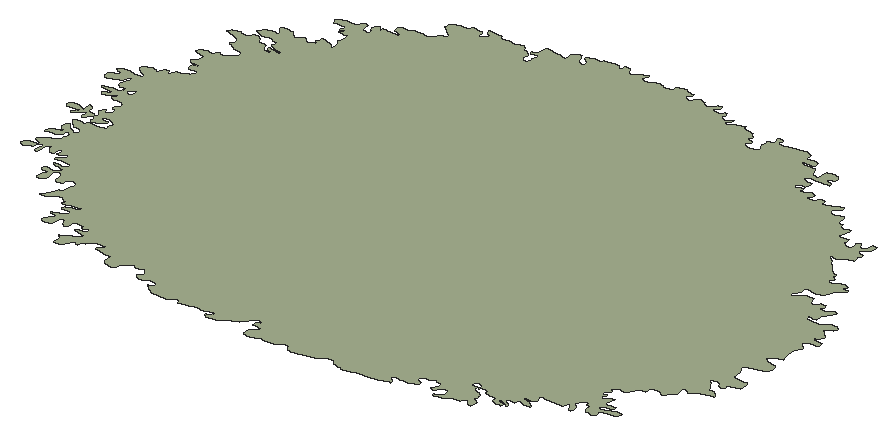
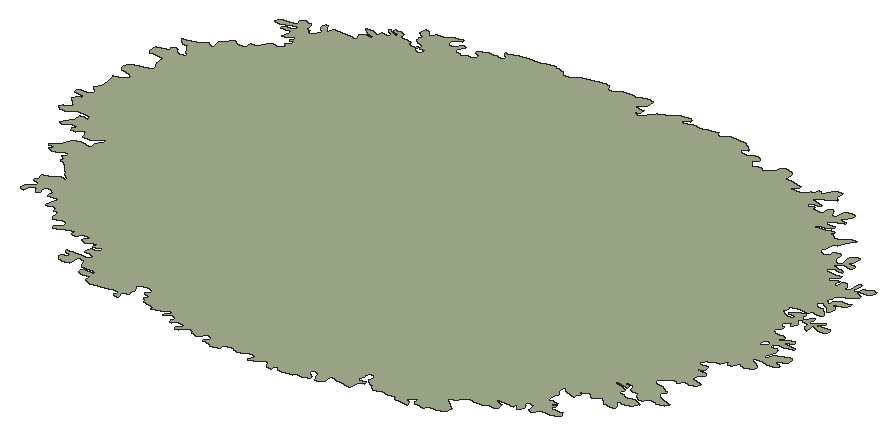
# SketchUp Ruby script. Lengths in inches.
U = 1.inch
M = Sketchup.active_model
def pt(a) = Geom::Point3d.new(a.map { |v| v * U })
def face(e, loops, mat)
  f = e.add_face(loops[0].map { |a| pt(a) })
  loops[1..].each { |l| e.add_face(l.map { |a| pt(a) }).erase! }
  f.material = f.back_material = mat if mat
  f
end
# faces: each face lists its corners as indices into pts; further lists are holes
def faces(e, pts, list, mat = nil) = list.each { |f| face(e, (f[0].is_a?(Array) ? f : [f]).map { |l| l.map { |i| pts[i] } }, mat) }
# xy, xz, yz: faces in a plane at the given z, y or x. An outline is a flat list of corners, or four numbers for a rectangle; further outlines are holes
def ring(l) = l.size == 4 ? [[l[0], l[1]], [l[2], l[1]], [l[2], l[3]], [l[0], l[3]]] : l.each_slice(2).to_a
def flat(e, list, mat, &to3) = list.each { |f| face(e, (f[0].is_a?(Array) ? f : [f]).map { |l| ring(l).map { |u, v| to3.(u, v) } }, mat) }
def xy(e, z, list, mat = nil) = flat(e, list, mat) { |x, y| [x, y, z] }
def xz(e, y, list, mat = nil) = flat(e, list, mat) { |x, z| [x, y, z] }
def yz(e, x, list, mat = nil) = flat(e, list, mat) { |y, z| [x, y, z] }
def lines(e, pts, list) = list.each { |a, b| e.add_line(pt(pts[a]), pt(pts[b])) }
# prism: a flat outline (further loops are holes) pulled along v
def prism(e, loops, v, mat = nil)
  f = face(e, loops, mat); d = Geom::Vector3d.new(v.map { |x| x * U })
  f.pushpull(f.normal.samedirection?(d) ? d.length : -d.length)
end
def box(e, o, s, mat = nil) = prism(e, [[o, [o[0] + s[0], o[1], o[2]], [o[0] + s[0], o[1] + s[1], o[2]], [o[0], o[1] + s[1], o[2]]]], [0, 0, s[2]], mat)
def at(x, y, z, deg = 0) = Geom::Transformation.translation(pt([x, y, z])) * Geom::Transformation.rotation(ORIGIN, Z_AXIS, deg.degrees)
def axes(o, x, y, z) = Geom::Transformation.new([*x, 0, *y, 0, *z, 0, *pt(o).to_a, 1])
def part(name) = M.definitions.add(name)
# library, detail: a bought-in or finely detailed component or shape, given as its bounding box
def library(name, o, s) = part(name).tap { |d| box(d.entities, o, s) }
def detail(e, o, s) = box(e.add_group.entities, o, s)
def put(e, d, t, mat = nil) = e.add_instance(d, t).tap { |i| i.material = mat if mat }
def group(e, t, mat = nil) = e.add_group.tap { |g| g.transformation = t; g.material = mat if mat }.entities
root = M.entities
M.materials.add("Boxwoodplan").color = [166, 177, 144]
xy(root,9.058,[[[52.292,67.129,52.181,67.133,52.086,67.159,52.03,67.215,52.028,67.317,52.054,67.382,52.118,67.445,52.167,67.509,52.225,67.606,52.039,67.635,51.949,67.644,51.969,67.732,52.055,67.79,52.086,67.8,52.081,67.846,51.992,67.877,51.876,67.837,51.779,67.706,51.636,67.551,51.475,67.464,51.37,67.441,51.309,67.416,51.293,67.373,51.149,67.281,50.955,67.251,50.866,67.26,50.786,67.306,50.786,67.328,50.831,67.359,50.922,67.437,50.99,67.483,50.901,67.498,50.788,67.48,50.668,67.436,50.572,67.445,50.475,67.454,50.378,67.447,50.251,67.403,50.051,67.356,49.962,67.349,49.924,67.443,49.916,67.465,49.849,67.473,49.76,67.454,49.591,67.336,49.391,67.328,49.161,67.353,48.994,67.446,48.853,67.61,49.036,67.702,48.936,67.756,48.8,67.772,48.674,67.749,48.602,67.697,48.521,67.672,48.405,67.738,48.363,67.806,48.451,67.847,48.477,67.907,48.482,67.957,48.441,68.009,48.369,68.085,48.283,68.117,48.196,68.064,48.13,68.038,48.074,68.08,48.057,68.103,48.033,68.121,48.004,68.111,47.924,68.058,47.853,68.01,47.777,67.923,47.765,67.79,47.694,67.749,47.644,67.723,47.584,67.725,47.485,67.746,47.398,67.793,47.354,67.861,47.346,67.951,47.355,68.018,47.368,68.04,47.349,68.08,47.135,68.1,47.203,68.135,47.177,68.136,47.084,68.13,46.914,68.146,46.837,68.173,46.82,68.206,46.835,68.224,46.96,68.314,46.958,68.371,46.873,68.393,46.714,68.39,46.583,68.319,46.486,68.233,46.411,68.199,46.364,68.172,46.363,68.154,46.399,68.101,46.383,68.046,46.313,68.081,46.249,68.121,46.188,68.072,46.166,68.017,46.134,67.904,46.087,67.855,46.014,67.822,45.923,67.816,45.853,67.841,45.834,67.874,45.841,67.892,45.862,67.932,45.884,67.991,45.853,68.048,45.752,68.149,45.866,68.229,45.927,68.269,46.007,68.285,46.074,68.315,46.129,68.37,46.214,68.476,46.142,68.503,46.0625,68.511,45.93,68.53,45.892,68.565,45.899,68.584,45.974,68.62,46.136,68.657,46.178,68.709,46.173,68.748,46.147,68.764,45.997,68.711,45.951,68.732,45.952,68.752,45.975,68.814,45.814,68.825,45.733,68.833,45.679,68.826,45.672,68.806,45.656,68.71,45.641,68.642,45.599,68.591,45.552,68.578,45.533,68.594,45.474,68.639,45.429,68.757,45.39,68.783,45.363,68.784,45.309,68.777,45.302,68.757,45.3,68.641,45.246,68.523,45.185,68.449,45.105,68.419,45.026,68.422,44.98,68.448,44.947,68.506,44.947,68.564,45.001,68.677,45.115,68.784,45.135,68.803,45.122,68.823,45.095,68.829,45.015,68.847,44.934,68.86,44.907,68.875,44.914,68.895,44.934,68.914,45.083,68.982,45.245,69.005,45.287,69.108,45.26,69.169,45.213,69.191,45.186,69.187,45.023,69.168,44.982,69.2,44.989,69.22,45.016,69.279,45.174,69.334,45.346,69.403,45.394,69.442,45.381,69.463,45.284,69.436,45.113,69.417,44.969,69.372,44.88,69.386,44.853,69.392,44.859,69.412,44.88,69.426,44.935,69.47,44.907,69.507,44.88,69.503,44.797,69.511,44.742,69.56,44.728,69.601,44.701,69.597,44.618,69.575,44.461,69.489,44.312,69.413,44.238,69.38,44.183,69.392,44.196,69.412,44.215,69.452,44.242,69.469,44.266,69.55,44.316,69.65,44.348,69.759,44.399,69.812,44.472,69.852,44.516,69.972,44.538,70.112,44.558,70.227,44.554,70.285,44.509,70.321,44.428,70.335,44.342,70.335,44.268,70.31,44.258,70.245,44.259,70.184,44.226,70.124,44.138,70.087,44.081,70.096,44.043,70.155,44.032,70.216,44.006,70.337,44.001,70.4,43.96,70.453,43.933,70.475,43.895,70.491,43.836,70.479,43.802,70.46,43.8,70.428,43.792,70.366,43.795,70.229,43.82,70.167,43.812,70.103,43.761,70.038,43.713,70.01,43.675,69.998,43.637,70.003,43.595,70.011,43.577,70.039,43.573,70.166,43.594,70.223,43.639,70.276,43.655,70.306,43.647,70.334,43.59,70.34,43.508,70.346,43.471,70.362,43.448,70.39,43.445,70.453,43.46,70.483,43.495,70.499,43.667,70.472,43.746,70.497,43.795,70.526,43.856,70.573,43.869,70.636,43.846,70.662,43.802,70.664,43.725,70.67,43.633,70.681,43.532,70.717,43.513,70.746,43.519,70.76,43.538,70.763,43.598,70.775,43.773,70.761,43.863,70.787,43.875,70.844,43.849,70.907,43.777,70.946,43.698,70.953,43.585,70.946,43.485,70.921,43.402,70.939,43.398,70.968,43.418,70.997,43.465,71.054,43.531,71.11,43.584,71.19,43.576,71.224,43.531,71.241,43.466,71.24,43.348,71.14,43.308,71.141,43.274,71.161,43.296,71.22,43.312,71.287,43.269,71.35,43.229,71.366,43.209,71.367,43.203,71.352,43.207,71.306,43.204,71.164,43.163,71.102,43.124,71.108,43.089,71.131,42.991,71.262,42.967,71.327,42.942,71.355,42.927,71.344,42.871,71.293,42.836,71.234,42.856,71.103,42.861,71.037,42.841,70.971,42.791,70.962,42.757,70.978,42.747,71.023,42.767,71.155,42.776,71.233,42.776,71.27,42.761,71.282,42.746,71.272,42.667,71.237,42.627,71.183,42.618,71.12,42.579,71.077,42.442,70.987,42.402,70.977,42.358,70.986,42.278,71.026,42.258,71.056,42.262,71.089,42.295,71.151,42.392,71.237,42.482,71.263,42.572,71.263,42.667,71.267,42.606,71.318,42.455,71.404,42.438,71.466,42.491,71.503,42.583,71.573,42.702,71.635,42.82,71.709,42.856,71.723,42.882,71.746,42.908,71.789,42.911,71.882,42.944,72.003,42.945,72.065,42.924,72.086,42.902,72.095,42.839,72.109,42.806,72.104,42.802,72.088,42.814,71.996,42.772,71.934,42.724,71.899,42.647,71.871,42.576,71.858,42.415,71.833,42.38,71.839,42.367,71.853,42.367,71.86,42.376,71.901,42.393,71.947,42.435,71.995,42.504,72.042,42.563,72.063,42.621,72.065,42.66,72.068,42.68,72.075,42.703,72.096,42.698,72.121,42.644,72.151,42.576,72.207,42.544,72.264,42.54,72.331,42.553,72.382,42.605,72.426,42.631,72.432,42.642,72.425,42.662,72.411,42.705,72.35,42.754,72.304,42.882,72.226,42.956,72.192,42.991,72.177,43.011,72.184,43.035,72.206,43.042,72.222,43.053,72.263,43.038,72.32,42.995,72.366,42.963,72.389,42.929,72.401,42.869,72.401,42.795,72.404,42.752,72.446,42.666,72.519,42.607,72.569,42.568,72.617,42.569,72.646,42.593,72.671,42.649,72.698,42.684,72.703,42.725,72.7,42.785,72.679,42.847,72.677,42.883,72.684,42.917,72.726,42.966,72.757,43.025,72.764,43.096,72.764,43.25,72.771,43.39,72.792,43.423,72.808,43.424,72.826,43.418,72.868,43.406,72.913,43.417,72.957,43.447,73.06,43.434,73.083,43.411,73.097,43.354,73.126,43.301,73.164,43.228,73.192,43.155,73.195,43.105,73.184,43.084,73.17,43.059,73.119,43.064,73.098,43.075,73.093,43.099,73.088,43.25,73.076,43.276,73.071,43.281,73.0625,43.272,73.046,43.232,73.007,43.187,72.964,43.122,72.928,43.06,72.884,42.988,72.849,42.951,72.852,42.931,72.863,42.906,72.9,42.899,72.995,42.882,73.02,42.9,73.034,42.906,73.077,42.9,73.088,42.889,73.088,42.874,73.087,42.848,73.083,42.816,73.076,42.798,73.065,42.717,72.97,42.685,72.915,42.654,72.892,42.631,72.895,42.605,72.916,42.596,72.932,42.59,72.973,42.619,73.057,42.624,73.102,42.615,73.13,42.595,73.137,42.557,73.128,42.537,73.114,42.491,73.064,42.369,72.957,42.333,72.932,42.307,72.927,42.27,72.935,42.258,72.951,42.349,73.057,42.412,73.102,42.426,73.129,42.425,73.145,42.416,73.152,42.405,73.148,42.39,73.143,42.359,73.131,42.275,73.108,42.108,73.089,42.035,73.096,41.987,73.121,41.965,73.149,41.964,73.165,41.981,73.217,42.029,73.264,42.089,73.281,42.16,73.284,42.234,73.266,42.362,73.223,42.448,73.197,42.459,73.201,42.459,73.22,42.45,73.239,42.425,73.287,42.424,73.342,42.431,73.407,42.443,73.437,42.46,73.45,42.509,73.413,42.548,73.363,42.575,73.317,42.585,73.255,42.597,73.204,42.612,73.176,42.635,73.175,42.77,73.157,42.843,73.144,42.878,73.14,42.896,73.154,42.911,73.202,42.856,73.244,42.797,73.309,42.78,73.335,42.78,73.352,42.814,73.46,42.844,73.483,42.871,73.489,42.886,73.477,42.895,73.459,42.924,73.414,42.935,73.39,42.947,73.391,42.968,73.404,43.048,73.482,43.065,73.528,43.066,73.579,43.052,73.611,43.031,73.623,42.968,73.646,42.928,73.666,42.92,73.687,42.936,73.736,42.992,73.773,43.026,73.795,43.039,73.816,43.047,73.869,43.045,73.916,42.95,73.992,42.806,74.014,42.744,74.031,42.709,74.013,42.681,74.014,42.612,74.031,42.593,74.058,42.602,74.082,42.728,74.185,42.722,74.217,42.7,74.233,42.655,74.225,42.626,74.216,42.5,74.154,42.46,74.107,42.411,74.063,42.342,74.049,42.314,74.05,42.267,74.102,42.295,74.126,42.3125,74.165,42.344,74.188,42.438,74.22,42.483,74.25,42.472,74.281,42.459,74.283,42.449,74.276,42.423,74.27,42.384,74.273,42.249,74.284,42.102,74.3125,42.078,74.327,42.084,74.347,42.109,74.375,42.322,74.435,42.385,74.434,42.446,74.419,42.506,74.391,42.533,74.393,42.539,74.403,42.588,74.48,42.612,74.495,42.618,74.515,42.618,74.583,42.607,74.593,42.594,74.591,42.536,74.591,42.479,74.585,42.432,74.568,42.408,74.576,42.387,74.596,42.362,74.63,42.342,74.718,42.353,74.806,42.383,74.848,42.389,74.88,42.402,74.923,42.439,74.944,42.435,74.99,42.413,75.026,42.324,75.003,42.306,74.969,42.307,74.95,42.31,74.886,42.23,74.839,42.089,74.745,41.933,74.7,41.849,74.725,41.807,74.778,41.798,74.904,41.926,74.99,42.009,75.003,42.052,75.027,42.076,75.061,42.075,75.081,41.989,75.112,41.916,75.138,41.854,75.194,41.889,75.249,41.965,75.278,42.061,75.312,42.126,75.311,42.305,75.267,42.397,75.246,42.482,75.25,42.533,75.269,42.539,75.289,42.523,75.355,42.462,75.407,42.417,75.415,42.305,75.485,42.258,75.527,42.244,75.564,42.237,75.617,42.237,75.644,42.25,75.659,42.292,75.695,42.343,75.709,42.457,75.741,42.488,75.751,42.528,75.75,42.578,75.746,42.591,75.733,42.606,75.703,42.62,75.689,42.63,75.689,42.658,75.692,42.674,75.704,42.695,75.754,42.723,75.787,42.739,75.81,42.742,75.835,42.758,75.86,42.778,75.872,42.826,75.884,42.865,75.877,42.886,75.833,42.89,75.781,42.907,75.755,42.928,75.754,42.97,75.796,42.995,75.838,43.009,75.942,43.025,75.968,43.057,75.975,43.089,75.974,43.108,75.963,43.129,75.94,43.161,75.94,43.214,75.961,43.258,76.007,43.272,76.032,43.261,76.046,43.321,76.043,43.35,76.046,43.366,76.066,43.371,76.114,43.405,76.155,43.439,76.2,43.385,76.243,43.318,76.272,43.281,76.271,43.248,76.261,43.206,76.249,43.164,76.255,43.142,76.271,43.121,76.295,43.098,76.397,43.111,76.423,43.116,76.439,43.126,76.443,43.231,76.463,43.277,76.472,43.295,76.483,43.285,76.486,43.199,76.514,43.133,76.526,43.105,76.519,43.07,76.52,43.034,76.52,42.998,76.532,42.96,76.582,42.942,76.611,42.942,76.642,42.957,76.663,42.986,76.678,43.017,76.697,43.025,76.725,43.055,76.782,43.082,76.836,43.088,76.89,43.081,76.917,43.041,76.928,42.963,76.954,42.79,77.001,42.754,77.018,42.737,77.042,42.773,77.097,42.817,77.131,42.863,77.159,42.918,77.178,42.97,77.1875,43.023,77.184,43.078,77.16,43.133,77.162,43.16,77.167,43.173,77.187,43.19,77.228,43.227,77.264,43.248,77.282,43.274,77.284,43.343,77.267,43.405,77.256,43.431,77.253,43.455,77.268,43.542,77.336,43.629,77.401,43.683,77.498,43.679,77.542,43.638,77.579,43.521,77.617,43.395,77.647,43.309,77.719,43.251,77.755,43.182,77.776,43.155,77.788,43.141,77.808,43.163,77.855,43.211,77.896,43.209,77.981,43.159,78.06,43.029,78.116,42.741,78.212,42.72,78.246,42.792,78.31,42.913,78.362,43.018,78.367,43.075,78.353,43.119,78.327,43.168,78.317,43.221,78.326,43.282,78.337,43.311,78.368,43.326,78.448,43.343,78.483,43.397,78.482,43.454,78.471,43.502,78.451,43.569,78.392,43.593,78.358,43.607,78.318,43.608,78.249,43.614,78.245,43.623,78.249,43.65,78.262,43.701,78.268,43.79,78.271,43.87,78.235,43.904,78.17,43.929,78.092,43.999,78.047,44.039,78.035,44.057,78.034,44.084,78.043,44.179,78.05,44.196,78.055,44.176,78.071,44.113,78.095,44.061,78.099,44.023,78.118,44.004,78.152,44.001,78.164,44.004,78.184,44.019,78.191,44.054,78.192,44.096,78.185,44.202,78.156,44.317,78.152,44.369,78.159,44.387,78.162,44.413,78.173,44.369,78.203,44.328,78.213,44.242,78.228,44.184,78.242,44.143,78.244,44.121,78.248,44.096,78.263,44.044,78.289,43.997,78.315,43.975,78.348,43.985,78.404,44.014,78.442,44.055,78.471,44.015,78.502,43.96,78.517,43.917,78.52,43.862,78.528,43.831,78.555,43.813,78.591,43.799,78.6,43.77,78.599,43.654,78.571,43.602,78.557,43.553,78.559,43.505,78.562,43.456,78.578,43.408,78.595,43.368,78.602,43.282,78.65,43.307,78.662,43.309,78.669,43.32,78.709,43.336,78.745,43.362,78.782,43.393,78.814,43.437,78.839,43.49,78.862,43.535,78.873,43.641,78.867,43.718,78.862,43.751,78.858,43.762,78.857,43.762,78.87,43.754,78.912,43.733,78.956,43.697,78.995,43.654,79.026,43.621,79.073,43.623,79.096,43.634,79.117,43.681,79.147,43.733,79.17,43.76,79.169,43.786,79.163,43.84,79.148,43.908,79.142,43.955,79.127,43.979,79.114,43.997,79.095,44.041,79.055,44.08,79.02,44.125,78.989,44.181,78.976,44.235,78.981,44.28,79.01,44.312,79.046,44.361,79.084,44.387,79.083,44.409,79.069,44.45,79.027,44.497,78.994,44.625,79.019,44.699,79.037,44.74,79.065,44.746,79.085,44.725,79.102,44.674,79.124,44.664,79.147,44.672,79.169,44.688,79.214,44.695,79.273,44.699,79.299,44.722,79.315,44.749,79.316,44.779,79.308,44.821,79.288,44.955,79.248,45.016,79.226,45.055,79.193,45.082,79.153,45.097,79.13,45.104,79.123,45.113,79.126,45.121,79.131,45.154,79.176,45.16,79.212,45.15,79.315,45.128,79.362,45.104,79.397,45.069,79.436,45.059,79.466,45.07,79.477,45.081,79.475,45.103,79.476,45.102,79.484,45.107,79.508,45.1,79.549,45.085,79.705,45.087,79.782,44.972,79.802,44.875,79.804,44.8125,79.8125,44.795,79.819,44.781,79.83,44.794,79.839,44.907,79.882,44.941,79.911,44.94,79.924,44.917,79.948,44.881,79.952,44.828,79.94,44.78,79.918,44.763,79.919,44.748,79.945,44.774,80.028,44.777,80.069,44.776,80.082,44.752,80.103,44.663,80.085,44.55,80.088,44.441,80.105,44.38,80.185,44.378,80.213,44.416,80.25,44.512,80.303,44.561,80.33,44.615,80.335,44.74,80.332,44.831,80.337,44.891,80.346,44.931,80.384,44.971,80.418,44.979,80.461,45.005,80.5,45.061,80.513,45.098,80.509,45.141,80.475,45.152,80.389,45.159,80.3,45.183,80.257,45.238,80.231,45.33,80.212,45.385,80.234,45.403,80.276,45.38,80.319,45.333,80.355,45.277,80.442,45.313,80.521,45.387,80.603,45.406,80.606,45.43,80.576,45.449,80.528,45.523,80.447,45.551,80.421,45.542,80.475,45.524,80.57,45.58,80.587,45.641,80.582,45.768,80.578,45.881,80.575,46.003,80.557,46.021,80.557,46.009,80.587,45.958,80.629,45.828,80.681,45.79,80.689,45.767,80.735,45.769,80.826,45.804,80.871,45.853,80.896,45.969,80.901,46.066,80.91,46.161,80.977,46.287,80.982,46.403,80.971,46.499,80.953,46.62,80.946,46.663,80.991,46.676,81.038,46.719,81.133,46.808,81.187,46.928,81.244,46.94,81.26,46.923,81.294,46.882,81.332,46.775,81.413,46.707,81.487,46.649,81.528,46.592,81.57,46.623,81.577,46.622,81.591,46.617,81.612,46.606,81.679,46.609,81.709,46.644,81.744,46.727,81.785,46.81,81.821,46.848,81.827,46.904,81.826,46.991,81.816,47.014,81.808,47.038,81.81,47.07,81.843,47.122,81.918,47.158,81.932,47.215,81.936,47.317,81.93,47.413,81.898,47.445,81.877,47.474,81.835,47.475,81.765,47.478,81.736,47.483,81.715,47.506,81.704,47.559,81.715,47.604,81.745,47.666,81.798,47.691,81.822,47.712,81.834,47.725,81.85,47.64,81.897,47.602,81.913,47.559,81.956,47.534,82.036,47.535,82.067,47.593,82.083,47.785,82.055,47.882,82.039,47.917,82.026,47.917,81.98,47.927,81.952,47.987,81.948,48.091,81.962,48.193,81.975,48.235,81.971,48.282,81.957,48.309,81.934,48.334,81.933,48.359,81.943,48.503,81.972,48.544,81.981,48.596,81.987,48.632,81.984,48.677,81.957,48.707,81.886,48.733,81.863,48.778,81.844,48.818,81.833,48.858,81.808,48.91,81.753,48.964,81.696,48.951,81.619,48.944,81.545,48.958,81.515,48.989,81.485,49.016,81.461,49.063,81.453,49.099,81.45,49.144,81.481,49.157,81.512,49.158,81.553,49.146,81.628,49.183,81.787,49.172,81.817,49.154,81.829,49.13,81.833,49.091,81.834,49.039,81.828,49.003,81.826,48.956,81.835,48.931,81.858,48.938,81.88,48.966,81.896,49.005,81.91,49.05,81.937,49.075,82.013,49.079,82.178,49.079,82.21,49.102,82.228,49.128,82.233,49.227,82.222,49.426,82.201,49.517,82.19,49.606,82.169,49.693,82.153,49.744,82.147,49.739,82.355,49.807,82.427,49.892,82.486,49.946,82.477,49.974,82.441,50.022,82.37,50.045,82.297,50.053,82.26,50.051,82.241,50.078,82.206,50.183,82.173,50.235,82.173,50.274,82.204,50.277,82.279,50.174,82.36,50.096,82.419,50.108,82.453,50.152,82.49,50.246,82.541,50.296,82.55,50.377,82.538,50.481,82.537,50.504,82.615,50.714,82.643,50.814,82.661,50.922,82.647,51.001,82.578,51.034,82.543,51.061,82.541,51.101,82.568,51.099,82.643,51.09,82.685,51.103,82.72,51.153,82.729,51.208,82.715,51.279,82.621,51.3,82.548,51.333,82.513,51.382,82.498,51.433,82.503,51.479,82.53,51.567,82.613,51.648,82.668,51.75,82.715,51.798,82.7,51.812,82.663,51.76,82.592,51.734,82.557,51.742,82.515,51.831,82.457,51.931,82.443,51.981,82.452,52.031,82.498,52.109,82.566,52.224,82.581,52.339,82.553,52.37,82.523,52.447,82.492,52.547,82.511,52.629,82.565,52.629,82.678,52.686,82.721,52.799,82.745,52.904,82.74,52.985,82.681,53.131,82.66,53.185,82.651,53.191,82.614,53.117,82.546,53.084,82.473,53.096,82.437,53.168,82.396,53.27,82.401,53.323,82.433,53.343,82.472,53.363,82.544,53.412,82.567,53.436,82.579,53.487,82.579,53.59,82.541,53.633,82.47,53.719,82.417,53.849,82.447,53.884,82.478,53.89,82.52,53.93,82.603,54.037,82.622,54.067,82.592,54.073,82.55,54.02,82.466,53.972,82.448,53.945,82.413,54.005,82.349,54.136,82.337,54.227,82.373,54.294,82.444,54.319,82.45,54.328,82.433,54.346,82.392,54.37,82.357,54.359,82.301,54.339,82.257,54.357,82.222,54.446,82.179,54.554,82.184,54.609,82.203,54.66,82.258,54.677,82.273,54.679,82.255,54.666,82.212,54.593,82.132,54.559,82.102,54.57,82.066,54.617,82.047,54.675,82.048,54.771,82.088,54.853,82.146,55.073,82.225,55.095,82.153,55.118,82.123,55.169,82.118,55.285,82.11,55.409,82.084,55.424,82.013,55.447,81.983,55.493,81.964,55.516,81.93,55.502,81.892,55.475,81.795,55.592,81.773,55.638,81.755,55.648,81.72,55.574,81.65,55.56,81.613,55.576,81.579,55.652,81.527,55.755,81.5,55.856,81.496,55.968,81.563,56.01,81.639,55.952,81.71,55.919,81.779,55.939,81.885,55.948,81.922,55.919,81.956,55.915,81.992,55.957,82.018,56.058,82.022,56.047,82.122,56.005,82.274,56.055,82.287,56.12,82.275,56.173,82.256,56.204,82.199,56.154,82.131,56.158,82.095,56.204,82.076,56.312,82.076,56.442,82.111,56.949,82.178,56.995,82.168,57.041,82.145,57.087,82.121,57.121,82.097,57.152,82.027,57.135,81.935,57.339,81.949,57.404,81.943,57.489,81.911,57.526,81.805,57.511,81.757,57.495,81.724,57.454,81.717,57.284,81.749,57.22,81.755,57.177,81.755,57.157,81.749,57.154,81.733,57.182,81.685,57.223,81.666,57.27,81.666,57.443,81.681,57.512,81.683,57.596,81.648,57.633,81.609,57.664,81.546,57.732,81.437,57.811,81.398,57.896,81.394,57.927,81.435,57.921,81.518,57.903,81.571,57.91,81.637,57.951,81.687,58.052,81.719,58.161,81.732,58.25,81.701,58.298,81.659,58.332,81.597,58.333,81.551,58.271,81.495,58.205,81.482,58.164,81.471,58.132,81.437,58.136,81.407,58.185,81.389,58.283,81.363,58.354,81.339,58.374,81.306,58.362,81.275,58.308,81.247,58.221,81.24,58.059,81.233,57.972,81.222,57.883,81.256,57.819,81.269,57.737,81.251,57.681,81.208,57.679,81.143,57.737,81.103,57.824,81.081,57.91,81.066,57.957,81.066,57.991,81.046,58.012,81.003,57.995,80.938,57.96,80.89,57.932,80.866,57.887,80.854,57.745,80.834,57.725,80.829,57.716,80.784,57.72,80.751,57.765,80.732,57.832,80.731,57.873,80.731,57.923,80.746,57.986,80.778,58,80.712,57.971,80.665,57.964,80.635,58.003,80.617,58.064,80.622,58.146,80.67,58.202,80.711,58.23,80.736,58.268,80.721,58.332,80.704,58.401,80.651,58.397,80.603,58.354,80.537,58.321,80.472,58.339,80.448,58.386,80.445,58.462,80.456,58.544,80.495,58.583,80.554,58.655,80.597,58.715,80.609,58.752,80.601,58.77,80.577,58.773,80.548,58.756,80.521,58.728,80.497,58.73,80.483,58.751,80.481,58.923,80.499,59.004,80.51,59.071,80.552,59.113,80.589,59.192,80.614,59.289,80.619,59.312,80.595,59.315,80.566,59.155,80.349,59.17,80.304,59.227,80.251,59.31,80.237,59.399,80.255,59.467,80.283,59.552,80.305,59.617,80.213,59.653,79.999,59.655,79.985,59.691,79.974,59.775,79.996,59.786,79.918,59.81,79.871,59.886,79.861,60.023,79.896,60.091,79.893,60.106,79.839,60.038,79.619,60.027,79.567,60.05,79.514,60.116,79.486,60.184,79.496,60.32,79.523,60.34,79.419,60.335,79.316,60.457,79.247,60.59,79.216,60.62,79.318,60.61,79.421,60.587,79.474,60.615,79.525,60.684,79.535,60.723,79.482,60.745,79.429,60.793,79.395,60.87,79.418,60.924,79.467,60.948,79.583,60.952,79.636,61.013,79.659,61.07,79.631,61.1,79.577,61.075,79.455,60.96,79.375,60.907,79.339,60.886,79.282,60.866,79.231,60.889,79.186,61.021,79.161,61.077,79.134,61.082,79.083,61.009,78.997,61.044,78.895,61.073,78.844,61.061,78.794,60.927,78.768,60.826,78.729,60.722,78.658,60.671,78.623,60.605,78.626,60.541,78.659,60.509,78.667,60.483,78.643,60.527,78.549,60.646,78.483,60.693,78.445,60.69,78.396,60.775,78.32,60.941,78.132,61.073,78.05,61.136,78.035,61.173,77.992,61.158,77.898,61.274,77.834,61.211,77.749,61.191,77.697,61.189,77.673,61.22,77.661,61.357,77.679,61.492,77.755,61.622,77.768,61.747,77.734,61.75,77.687,61.684,77.66,61.658,77.644,61.672,77.62,61.75,77.599,61.822,77.596,61.854,77.595,61.867,77.571,61.779,77.482,61.613,77.322,61.589,77.232,61.585,77.187,61.557,77.142,61.464,77.067,61.336,77.038,61.211,77.043,61.102,77.082,61.033,77.076,61.006,77.004,61.033,76.894,61.004,76.787,60.886,76.72,60.914,76.62,61.052,76.642,61.224,76.833,61.451,76.815,61.527,76.605,61.572,76.595,61.654,76.618,61.741,76.723,61.879,76.735,61.917,76.635,61.867,76.574,61.852,76.539,61.929,76.501,62.068,76.531,62.1875,76.598,62.234,76.614,62.324,76.592,62.302,76.477,62.191,76.384,62.126,76.289,62.134,76.113,62.12,76.078,62.027,76.056,61.895,76.087,61.92,75.981,62.051,75.941,62.197,75.936,62.346,75.965,62.583,76.087,62.719,76.099,62.811,76.008,62.778,75.905,62.638,75.849,62.591,75.825,62.5625,75.766,62.666,75.675,62.817,75.515,62.784,75.414,62.668,75.359,62.632,75.335,62.67,75.274,62.814,75.269,62.944,75.247,62.956,75.145,62.883,75.089,62.75,75.078,62.625,75.041,62.582,74.942,62.75,74.761,62.643,74.568,62.646,74.388,62.7,74.176,62.744,74.078,62.612,74.051,62.489,74.008,62.395,73.931,62.368,73.869,62.479,73.801,62.731,73.744,62.808,73.662,62.829,73.559,62.787,73.467,62.672,73.394,62.211,73.234,62.213,73.141,62.257,73.048,62.311,72.954,62.3125,72.863,62.307,72.803,62.304,72.773,62.33,72.719,62.451,72.676,62.576,72.672,62.702,72.682,62.744,72.68,62.802,72.633,62.813,72.453,62.786,72.395,62.677,72.347,62.55,72.33,62.509,72.331,62.463,72.281,62.505,72.191,62.492,72.163,62.407,72.144,62.366,72.145,62.296,72.17,62.264,72.26,62.194,72.292,62.071,72.297,62.029,72.291,62.013,72.233,62.089,72.156,62.176,71.992,62.204,71.969,62.23,71.918,62.248,71.888,62.329,71.877,62.409,71.86,62.494,71.792,62.557,71.71,62.554,71.681,62.47,71.656,62.221,71.616,62.026,71.488,61.953,71.469,61.858,71.544,61.818,71.553,61.754,71.52,61.757,71.435,61.813,71.27,61.771,71.264,61.738,71.219,61.689,71.18,61.635,71.066,61.596,71.019,61.562,71,61.526,71.013,61.404,71.1,61.341,71.115,61.298,71.116,61.253,71.098,61.19,71.063,61.16,70.991,61.17,70.938,61.152,70.874,60.99,70.852,60.938,70.81,60.906,70.759,60.859,70.718,60.847,70.655,60.816,70.609,60.782,70.583,60.745,70.573,60.676,70.564,60.578,70.575,60.518,70.55,60.456,70.502,60.426,70.457,60.501,70.419,60.528,70.376,60.492,70.32,60.437,70.284,60.416,70.225,60.415,70.209,60.414,70.194,60.433,70.186,60.505,70.18,60.531,70.182,60.551,70.182,60.555,70.166,60.517,70.097,60.498,70.049,60.495,70.02,60.536,70.018,60.675,70.094,60.744,70.11,60.825,70.107,60.809,70.004,60.791,69.89,60.791,69.843,60.814,69.82,60.854,69.818,60.918,69.845,60.999,69.846,61.058,69.832,61.098,69.827,61.104,69.798,61.064,69.76,60.985,69.73,60.919,69.722,60.836,69.696,60.797,69.658,60.78,69.602,60.784,69.587,60.824,69.586,60.906,69.611,61.064,69.673,61.218,69.703,61.344,69.705,61.396,69.685,61.371,69.611,61.35,69.569,61.289,69.518,61.136,69.492,60.997,69.491,60.936,69.482,60.905,69.427,60.931,69.308,60.916,69.264,60.835,69.243,60.699,69.255,60.641,69.261,60.597,69.314,60.588,69.426,60.588,69.468,60.576,69.496,60.567,69.511,60.547,69.512,60.489,69.525,60.484,69.581,60.486,69.595,60.482,69.61,60.463,69.614,60.383,69.617,60.326,69.591,60.281,69.536,60.244,69.499,60.219,69.44,60.23,69.391,60.286,69.354,60.361,69.254,60.357,69.155,60.348,69.115,60.341,69.088,60.31,69.066,60.29,69.067,60.269,69.098,60.24,69.157,60.175,69.258,60.134,69.298,60.12,69.312,60.109,69.299,60.102,69.271,60.099,69.227,60.08,69.173,60.074,69.16,60.044,69.144,59.961,69.137,59.82,69.139,59.534,69.14,59.476,69.162,59.389,69.173,59.37,69.163,59.364,69.133,59.414,69.074,59.439,68.976,59.433,68.936,59.401,68.896,59.377,68.889,59.317,68.88,59.214,68.88,59.116,68.884,59.068,68.853,59.123,68.829,59.224,68.814,59.332,68.78,59.407,68.726,59.488,68.654,59.47,68.629,59.409,68.614,59.308,68.621,59.271,68.63,59.22,68.65,59.172,68.684,59.122,68.708,59.087,68.63,59.077,68.558,59.037,68.545,58.981,68.558,58.936,68.589,58.923,68.6,58.905,68.608,58.893,68.59,58.859,68.513,58.861,68.485,58.894,68.448,58.986,68.416,59.025,68.383,59.038,68.34,59.036,68.326,59.017,68.323,58.974,68.36,58.894,68.409,58.801,68.427,58.744,68.429,58.732,68.415,58.753,68.39,58.867,68.347,58.904,68.335,58.927,68.292,58.923,68.264,58.922,68.251,58.879,68.249,58.766,68.26,58.661,68.295,58.626,68.325,58.617,68.371,58.616,68.441,58.565,68.461,58.506,68.442,58.406,68.449,58.307,68.467,58.28,68.489,58.255,68.526,58.259,68.568,58.265,68.583,58.227,68.591,58.133,68.616,58.076,68.619,58.041,68.606,58.029,68.577,58.009,68.571,57.982,68.597,57.979,68.612,58.009,68.635,58.025,68.646,58.017,68.671,57.93,68.729,57.893,68.752,57.874,68.756,57.833,68.736,57.793,68.716,57.773,68.71,57.762,68.681,57.785,68.59,57.88,68.587,57.919,68.582,57.949,68.541,57.942,68.513,57.936,68.499,57.944,68.471,58.055,68.434,58.143,68.396,58.204,68.338,58.221,68.3125,58.22,68.299,58.185,68.283,58.165,68.273,58.196,68.251,58.251,68.225,58.263,68.2,58.212,68.168,58.2,68.141,58.225,68.106,58.31,68.062,58.388,67.994,58.387,67.851,58.366,67.825,58.314,67.814,58.26,67.829,58.222,67.874,58.182,67.939,58.164,67.949,58.126,67.944,58.074,67.926,58.052,67.897,58.053,67.854,58.052,67.84,58.019,67.828,57.842,67.819,57.834,67.826,57.786,67.808,57.742,67.777,57.658,67.692,57.606,67.661,57.532,67.651,57.394,67.643,57.34,67.658,57.338,67.698,57.447,67.762,57.547,67.834,57.544,67.937,57.538,67.98,57.538,67.994,57.507,68.015,57.447,68.034,57.373,68.034,57.289,67.95,57.269,67.911,57.212,67.866,57.197,67.857,57.161,67.865,57.124,67.88,57.112,67.907,57.152,67.999,57.212,68.094,57.213,68.135,57.145,68.189,57.034,68.224,56.982,68.246,56.945,68.238,56.92,68.215,56.886,68.171,56.853,68.156,56.811,68.157,56.755,68.166,56.718,68.168,56.68,68.145,56.599,68.05,56.613,68.01,56.687,67.97,56.742,67.938,56.769,67.917,56.778,67.89,56.754,67.851,56.694,67.807,56.592,67.756,56.537,67.735,56.464,67.738,56.409,67.76,56.335,67.769,56.29,67.745,56.253,67.743,56.221,67.76,56.166,67.766,56.093,67.752,56.071,67.717,56.081,67.659,56.178,67.575,56.205,67.536,56.206,67.51,56.206,67.497,56.188,67.492,55.898,67.391,55.623,67.369,55.39,67.373,55.299,67.371,55.177,67.31,55.074,67.275,54.977,67.279,54.939,67.281,54.89,67.299,54.842,67.328,54.781,67.325,54.692,67.334,54.608,67.376,54.548,67.433,54.517,67.478,54.458,67.491,54.359,67.479,54.263,67.438,54.183,67.398,54.084,67.325,53.987,67.269,53.894,67.24,53.653,67.222,53.463,67.186,53.366,67.19,53.301,67.284,53.27,67.351,53.182,67.365,53.091,67.352,52.995,67.28,52.93,67.217,52.84,67.21,52.663,67.233,52.478,67.24,52.4,67.189],[42.8,74.415,42.842,74.419,42.862,74.422,42.888,74.431,42.9,74.474,42.901,74.513,42.908,74.597,42.9,74.631,42.888,74.643,42.888,74.658,42.845,74.635,42.789,74.612,42.769,74.606,42.753,74.59,42.732,74.557,42.722,74.52,42.724,74.476,42.743,74.437,42.762,74.421]]],"Boxwoodplan")
